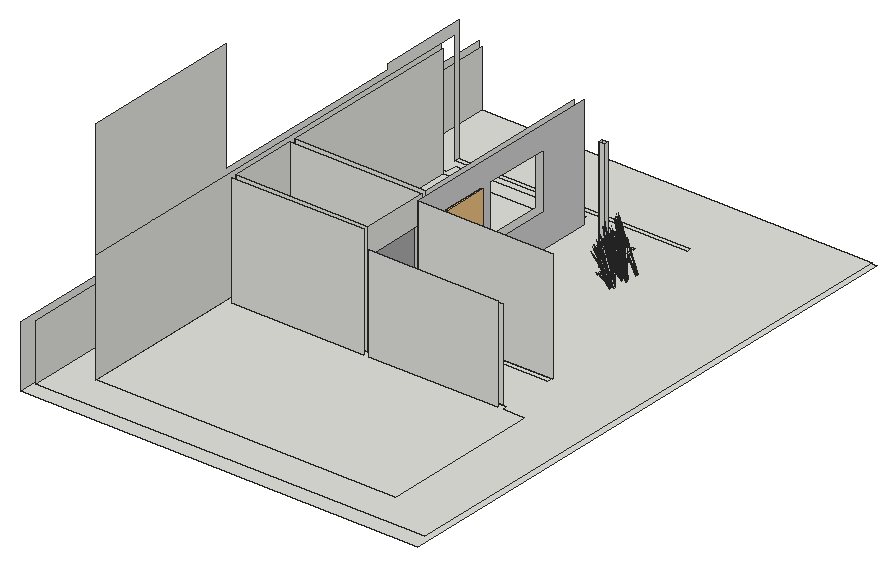
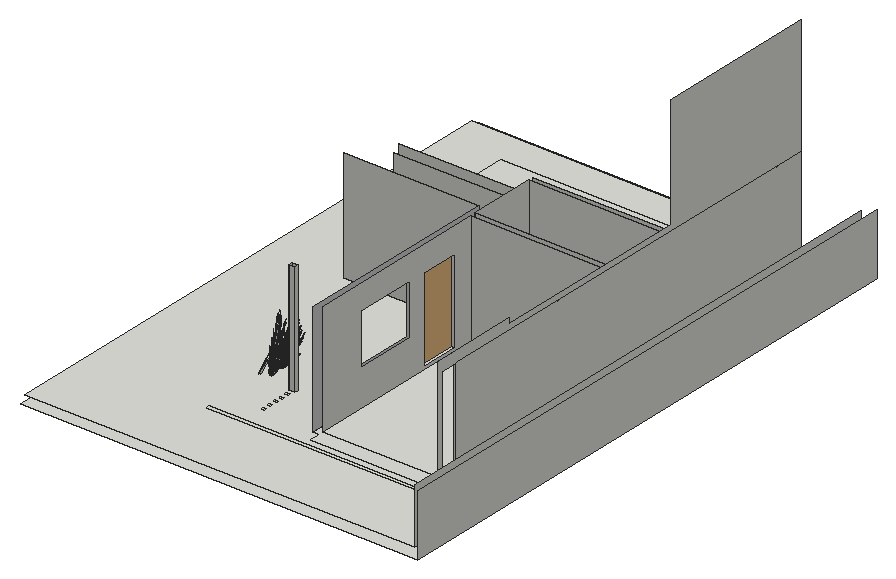
# SketchUp Ruby script. Lengths in inches.
U = 1.inch
M = Sketchup.active_model
def pt(a) = Geom::Point3d.new(a.map { |v| v * U })
def face(e, loops, mat)
  f = e.add_face(loops[0].map { |a| pt(a) })
  loops[1..].each { |l| e.add_face(l.map { |a| pt(a) }).erase! }
  f.material = f.back_material = mat if mat
  f
end
# faces: each face lists its corners as indices into pts; further lists are holes
def faces(e, pts, list, mat = nil) = list.each { |f| face(e, (f[0].is_a?(Array) ? f : [f]).map { |l| l.map { |i| pts[i] } }, mat) }
# xy, xz, yz: faces in a plane at the given z, y or x. An outline is a flat list of corners, or four numbers for a rectangle; further outlines are holes
def ring(l) = l.size == 4 ? [[l[0], l[1]], [l[2], l[1]], [l[2], l[3]], [l[0], l[3]]] : l.each_slice(2).to_a
def flat(e, list, mat, &to3) = list.each { |f| face(e, (f[0].is_a?(Array) ? f : [f]).map { |l| ring(l).map { |u, v| to3.(u, v) } }, mat) }
def xy(e, z, list, mat = nil) = flat(e, list, mat) { |x, y| [x, y, z] }
def xz(e, y, list, mat = nil) = flat(e, list, mat) { |x, z| [x, y, z] }
def yz(e, x, list, mat = nil) = flat(e, list, mat) { |y, z| [x, y, z] }
def lines(e, pts, list) = list.each { |a, b| e.add_line(pt(pts[a]), pt(pts[b])) }
# prism: a flat outline (further loops are holes) pulled along v
def prism(e, loops, v, mat = nil)
  f = face(e, loops, mat); d = Geom::Vector3d.new(v.map { |x| x * U })
  f.pushpull(f.normal.samedirection?(d) ? d.length : -d.length)
end
def box(e, o, s, mat = nil) = prism(e, [[o, [o[0] + s[0], o[1], o[2]], [o[0] + s[0], o[1] + s[1], o[2]], [o[0], o[1] + s[1], o[2]]]], [0, 0, s[2]], mat)
def at(x, y, z, deg = 0) = Geom::Transformation.translation(pt([x, y, z])) * Geom::Transformation.rotation(ORIGIN, Z_AXIS, deg.degrees)
def axes(o, x, y, z) = Geom::Transformation.new([*x, 0, *y, 0, *z, 0, *pt(o).to_a, 1])
def part(name) = M.definitions.add(name)
# library, detail: a bought-in or finely detailed component or shape, given as its bounding box
def library(name, o, s) = part(name).tap { |d| box(d.entities, o, s) }
def detail(e, o, s) = box(e.add_group.entities, o, s)
def put(e, d, t, mat = nil) = e.add_instance(d, t).tap { |i| i.material = mat if mat }
def group(e, t, mat = nil) = e.add_group.tap { |g| g.transformation = t; g.material = mat if mat }.entities
root = M.entities
M.materials.add("LightPink_Translucent").color = [144, 107, 117]
M.materials["LightPink_Translucent"].alpha = 0.75
M.materials.add("[0132_LightGray]").color = [169, 169, 169]
M.materials.add("[Cladding_Siding_White]1").color = [207, 207, 207]
c1 = library("porta+4",[0.2,-5.42,1.33],[46.55,4.72,83.21])
c2 = part("blade")
p = [[2.15,0.21,22],[0,0.17,0],[0.09,0.45,0],[2.18,0.31,22],[2.29,0.31,22],[0.38,0.45,0],
  [2.48,0.24,33],[2.49,0.24,33],[2.48,0.22,33]]
faces(c2.entities,p,[[0,1,2,3],[4,5,2,3],[6,3,4,7],[8,0,3,6]])
c3 = part("seeds")
p = [[0.3,-0.1,1.38],[-0.01,-0.03,1.59],[-0.01,-0.03,0.03],[0.14,-0.07,-0.07],[0.29,-0.03,3],[0.15,0.01,3.11]]
faces(c3.entities,p,[[0,1,2,3],[1,0,4,5]],"LightPink_Translucent")
c4 = part("blade with seeds")
put(c4.entities,c2,at(0,0,0))
put(c4.entities,c3,axes([2.4,0.25,30.99],[1.5799,-0.05474,1.17369],[-0.12525,1.92788,0.29478],[-0.07173,-0.02425,1.56792]))
xy(root,-6,[[0,0,426,612.89]])
xy(root,0,[[[9,9,426,606.89],[45,45,45,507,51,507,51,519,192,519,192,507,198,507,198,285,342,285,342,279,198,279,198,225,342,225,342,219,366,219,366,45],[45,525,294,531],[252,499,258,503],[252,491,258,495],[252,483,258,487],[252,475,258,479],[252,467,258,471],[252,459,258,463]],[51,225,192,297],[51,303,192,501]])
xy(root,3,[[192,324,198,366]])
xz(root,219,[[51,0,192,120],[198,0,336,102]])
xz(root,225,[[51,0,192,120],[198,0,336,96]])
xz(root,285,[[198,0,342,120]])
xz(root,297,[[51,0,192,120]])
xz(root,303,[[51,0,192,120]])
xz(root,324,[[192,3,198,93]])
xz(root,366,[[192,3,198,93]])
xz(root,459,[[252,0,258,120]])
xz(root,463,[[252,0,258,120]])
yz(root,0,[[0,-6,612.89,60]])
yz(root,9,[[9,0,606.89,60]])
yz(root,45,[[45,0,507,120],[525,0,525,120,45,120,45,246,219,246,219,126,435,126,435,132,531,132,531,0]])
yz(root,51,[[225,0,297,120],[303,0,501,120]])
yz(root,192,[[225,0,297,120],[[303,0,501,120],[324,3,366,93],[384,39,450,93]]])
yz(root,198,[[279,0,285,96],[[321,0,369,96],[324,3,366,93]]])
yz(root,198,[[225,0,279,96]],"[0132_LightGray]")
yz(root,198,[[[285,0,321,0,321,96,369,96,369,0,507,0,507,120,285,120],[381,36,453,96]]],"[Cladding_Siding_White]1")
yz(root,252,[[459,0,463,120]])
yz(root,258,[[459,0,463,120]])
put(root,c1,axes([195.24,320.8,-1.54],[0,1.02,0],[-1,0,0],[0,0,1.15408]))
put(root,c4,axes([282.74,451.66,3.875],[0.37107,-0.01478,1.71376],[-0.24616,0.64047,0.13857],[-0.5288,-0.03961,0.73262]))
put(root,c4,axes([282.9,452.79,3.875],[0.31041,-0.13801,1.71376],[0.26133,0.63772,0.13857],[-0.48731,0.14413,0.73262]))
put(root,c4,axes([281.93,453.875,2.59],[0.3109,0.05356,1.43002],[0.20038,0.54709,-0.30754],[-0.42231,0.10241,0.61141]))
put(root,c4,axes([284.68,452.125,3.34],[0.25429,-0.09438,1.77064],[0.08769,0.65901,0.13857],[-0.5508,0.08745,0.63284]))
put(root,c4,axes([284.1875,434.6,3.875],[0.37107,-0.01478,1.71376],[-0.24616,0.64047,0.13857],[-0.5288,-0.03961,0.73262]))
put(root,c4,axes([281.95,452.57,4.72],[-0.14609,0.08471,1.74944],[0.01243,0.61893,-0.27667],[-0.33486,0.08049,0.14031]))
put(root,c4,axes([283.85,451.07,4.98],[-0.89428,-0.01571,-0.71045],[0.06006,-0.66153,0.08574],[-0.37886,-0.06981,1.00501]))
put(root,c4,axes([283.13,451.23,2.59],[0.17466,0.18165,1.43002],[-0.40248,0.49377,-0.30754],[-0.41327,-0.11802,0.61141]))
put(root,c4,axes([282.42,452.21,4.53],[-0.74348,-0.18202,-0.35414],[0.21685,-0.53102,0.4572],[-0.29933,0.04869,0.87481]))
put(root,c4,axes([284.34,435.72,3.875],[0.31041,-0.13801,1.71376],[0.26133,0.63772,0.13857],[-0.48731,0.14413,0.73262]))
put(root,c4,axes([283.45,450.63,3.875],[0.3323,0.11241,1.71376],[-0.68769,0.4716,0.13857],[-0.42861,-0.21275,0.73262]))
put(root,c4,axes([283.375,436.81,2.59],[0.3109,0.05356,1.43002],[0.20038,0.54709,-0.30754],[-0.42231,0.10241,0.61141]))
put(root,c4,axes([280.33,453.19,4.71],[0.11417,0.0175,1.77383],[0.35319,0.57649,-0.16761],[-0.23371,0.15131,0.31391]))
put(root,c4,axes([282.93,452.48,4.68],[-0.24236,0.59349,-0.51099],[-0.83094,-0.20343,-0.3958],[-0.33455,0.05442,0.97773]))
put(root,c4,axes([283.56,451.2,4.68],[-0.6496,0.4322,-0.51099],[-0.5689,-0.45657,-0.3958],[-0.33005,-0.06576,0.97773]))
put(root,c4,axes([286.125,435.06,3.34],[0.25429,-0.09438,1.77064],[0.08769,0.65901,0.13857],[-0.5508,0.08745,0.63284]))
put(root,c4,axes([282.51,452.45,1.49],[0.02269,0.10283,1.76342],[-0.45738,0.53699,-0.26939],[-0.32488,-0.02707,0.30037]))
put(root,c4,axes([282.64,449.99,4.71],[0.06632,0.06511,1.77383],[-0.31973,0.58531,-0.16761],[-0.32381,0.00424,0.31391]))
put(root,c4,axes([281.28,455.02,2.77],[0.37283,-0.29571,1.1486],[0.14711,0.46813,0.84392],[-0.26943,0.08382,0.25299]))
put(root,c4,axes([283.38,449.6,4.72],[-0.19249,-0.00461,1.74944],[-0.61281,0.46055,-0.27667],[-0.32697,-0.0941,0.14031]))
put(root,c4,axes([283.39,435.5,4.72],[-0.14609,0.08471,1.74944],[0.01243,0.61893,-0.27667],[-0.33486,0.08049,0.14031]))
put(root,c4,axes([285.3,434,4.98],[-0.89428,-0.01571,-0.71045],[0.06006,-0.66153,0.08574],[-0.37886,-0.06981,1.00501]))
put(root,c4,axes([282.59,452.15,4.73],[0.25275,-0.59491,0.48003],[0.83094,0.20343,0.3958],[-0.32677,0.03575,0.9933]))
put(root,c4,axes([284.58,434.16,2.59],[0.17466,0.18165,1.43002],[-0.40248,0.49377,-0.30754],[-0.41327,-0.11802,0.61141]))
put(root,c4,axes([282.89,451.98,5.03],[0.45012,0.59081,-0.1216],[-0.79888,0.29033,-0.67495],[-0.33665,0.07795,1.02557]))
put(root,c4,axes([283.9,450.75,5.03],[-0.0479,0.66354,-0.1216],[-0.90696,-0.01814,-0.67495],[-0.3493,-0.04609,1.02557]))
put(root,c4,axes([283.32,450.79,4.53],[-0.50902,-0.40851,-0.35414],[0.58122,-0.38671,0.4572],[-0.29531,-0.05884,0.87481]))
put(root,c4,axes([282.53,451.99,4.73],[-0.32857,-0.44488,0.0643],[0.59916,-0.21775,0.50621],[-0.26412,0.04296,0.77189]))
put(root,c4,axes([283.86,435.15,4.53],[-0.74348,-0.18202,-0.35414],[0.21685,-0.53102,0.4572],[-0.29933,0.04869,0.87481]))
put(root,c4,axes([284.89,433.57,3.875],[0.3323,0.11241,1.71376],[-0.68769,0.4716,0.13857],[-0.42861,-0.21275,0.73262]))
put(root,c4,axes([284.03,453.22,3.875],[0.22344,-0.20048,1.71376],[0.56419,0.54113,0.13857],[-0.38697,0.24643,0.73262]))
put(root,c4,axes([282.69,453.74,4.53],[-0.77872,0.09325,-0.35414],[-0.20563,-0.53305,0.4572],[-0.22316,0.14318,0.87481]))
put(root,c4,axes([282.27,455.33,1.49],[0.12,0.06519,1.76342],[0.20347,0.60397,-0.26939],[-0.26596,0.12879,0.30037]))
put(root,c4,axes([282.09,451.77,2.77],[0.57115,-0.04669,1.1486],[-0.36229,0.41137,0.84392],[-0.28224,-0.06171,0.25299]))
put(root,c4,axes([281.77,436.125,4.71],[0.11417,0.0175,1.77383],[0.35319,0.57649,-0.16761],[-0.23371,0.15131,0.31391]))
put(root,c4,axes([284.37,435.42,4.68],[-0.24236,0.59349,-0.51099],[-0.83094,-0.20343,-0.3958],[-0.33455,0.05442,0.97773]))
put(root,c4,axes([285,434.13,4.68],[-0.6496,0.4322,-0.51099],[-0.5689,-0.45657,-0.3958],[-0.33005,-0.06576,0.97773]))
put(root,c4,axes([282.79,453.63,4.73],[-0.22187,-0.60049,0.48003],[0.87033,-0.10422,0.3958],[-0.25651,0.14123,0.9933]))
put(root,c4,axes([283.95,435.38,1.49],[0.02269,0.10283,1.76342],[-0.45738,0.53699,-0.26939],[-0.32488,-0.02707,0.30037]))
put(root,c4,axes([283.24,450.64,5.09],[0.7388,-0.48151,0.53763],[0.63717,0.51135,0.4433],[-0.34662,-0.08882,1.11249]))
put(root,c4,axes([282.62,453.51,4.73],[-0.61415,-0.2744,0.0643],[0.35756,-0.39076,0.50621],[-0.1969,0.12633,0.77189]))
put(root,c4,axes([284.08,432.92,4.71],[0.06632,0.06511,1.77383],[-0.31973,0.58531,-0.16761],[-0.32381,0.00424,0.31391]))
put(root,c4,axes([282.73,437.96,2.77],[0.37283,-0.29571,1.1486],[0.14711,0.46813,0.84392],[-0.26943,0.08382,0.25299]))
put(root,c4,axes([284.82,432.53,4.72],[-0.19249,-0.00461,1.74944],[-0.61281,0.46055,-0.27667],[-0.32697,-0.0941,0.14031]))
put(root,c4,axes([283.87,453.71,3.875],[0.16657,-0.22426,1.71376],[0.69879,0.4641,0.13857],[-0.31524,0.28926,0.73262]))
put(root,c4,axes([284.03,435.08,4.73],[0.25275,-0.59491,0.48003],[0.83094,0.20343,0.3958],[-0.32677,0.03575,0.9933]))
put(root,c4,axes([284.33,434.91,5.03],[0.45012,0.59081,-0.1216],[-0.79888,0.29033,-0.67495],[-0.33665,0.07795,1.02557]))
put(root,c4,axes([285.34,433.68,5.03],[-0.0479,0.66354,-0.1216],[-0.90696,-0.01814,-0.67495],[-0.3493,-0.04609,1.02557]))
put(root,c4,axes([284.76,433.73,4.53],[-0.50902,-0.40851,-0.35414],[0.58122,-0.38671,0.4572],[-0.29531,-0.05884,0.87481]))
put(root,c4,axes([283.2,452.15,5.05],[0.74348,0.18202,0.35414],[-0.21685,0.53102,-0.4572],[-0.29933,0.04869,0.87481]))
put(root,c4,axes([283.97,434.92,4.73],[-0.32857,-0.44488,0.0643],[0.59916,-0.21775,0.50621],[-0.26412,0.04296,0.77189]))
put(root,c4,axes([285.48,436.15,3.875],[0.22344,-0.20048,1.71376],[0.56419,0.54113,0.13857],[-0.38697,0.24643,0.73262]))
put(root,c4,axes([284.13,436.68,4.53],[-0.77872,0.09325,-0.35414],[-0.20563,-0.53305,0.4572],[-0.22316,0.14318,0.87481]))
put(root,c4,axes([283.33,453.81,4.68],[0.22982,0.59576,-0.51099],[-0.87033,0.10422,-0.3958],[-0.24941,0.16002,0.97773]))
put(root,c4,axes([283.58,450.64,4.73],[0.04505,-0.49615,0.0643],[0.68022,0.0136,0.50621],[-0.26056,-0.05192,0.77189]))
put(root,c4,axes([281.97,454.875,4.72],[-0.02224,0.12912,1.74944],[0.63107,0.44917,-0.27667],[-0.16521,0.21241,0.14031]))
put(root,c4,axes([283.71,438.26,1.49],[0.12,0.06519,1.76342],[0.20347,0.60397,-0.26939],[-0.26596,0.12879,0.30037]))
put(root,c4,axes([285.5,453.38,2.06],[-0.9306,-0.10697,-0.62353],[0.19638,-0.65984,-0.16365],[-0.27771,-0.07995,1.37633]))
put(root,c4,axes([283.54,434.71,2.77],[0.57115,-0.04669,1.1486],[-0.36229,0.41137,0.84392],[-0.28224,-0.06171,0.25299]))
put(root,c4,axes([285.67,449.78,5.43],[-0.59706,0.6255,-0.13619],[-0.86465,-0.36036,-0.75594],[-0.30056,-0.17672,1.14864]))
put(root,c4,axes([284.04,451.01,5.05],[0.50902,0.40851,0.35414],[-0.58122,0.38671,-0.4572],[-0.29531,-0.05884,0.87481]))
put(root,c4,axes([285.41,450.29,4.98],[-0.76283,-0.31537,-0.71045],[0.54213,-0.55263,0.08574],[-0.27638,-0.1883,1.00501]))
put(root,c4,axes([284.23,436.5625,4.73],[-0.22187,-0.60049,0.48003],[0.87033,-0.10422,0.3958],[-0.25651,0.14123,0.9933]))
put(root,c4,axes([285.05,450.3,4.68],[-0.88277,0.1551,-0.51099],[-0.15442,-0.58737,-0.3958],[-0.23711,-0.16832,0.97773]))
put(root,c4,axes([284.68,433.57,5.09],[0.7388,-0.48151,0.53763],[0.63717,0.51135,0.4433],[-0.34662,-0.08882,1.11249]))
put(root,c4,axes([284.0625,436.45,4.73],[-0.61415,-0.2744,0.0643],[0.35756,-0.39076,0.50621],[-0.1969,0.12633,0.77189]))
put(root,c4,axes([284.28,454.63,2.02],[-0.83726,-0.32623,-0.49651],[0.50045,-0.58498,0],[-0.19069,-0.0743,1.57504]))
put(root,c4,axes([283.91,449.77,1.49],[-0.08666,0.08595,1.76342],[-0.87574,0.18531,-0.26939],[-0.21156,-0.16858,0.30037]))
put(root,c4,axes([282.92,453.38,5.03],[0.82753,0.35977,-0.1216],[-0.47675,0.52101,-0.67495],[-0.2338,0.18111,1.02557]))
put(root,c4,axes([284.79,455.02,2.375],[-0.55932,0.6538,0],[-0.93577,-0.36461,-0.51607],[-0.21313,-0.08304,1.63711]))
put(root,c4,axes([285.31,436.65,3.875],[0.16657,-0.22426,1.71376],[0.69879,0.4641,0.13857],[-0.31524,0.28926,0.73262]))
put(root,c4,axes([284.64,435.09,5.05],[0.74348,0.18202,0.35414],[-0.21685,0.53102,-0.4572],[-0.29933,0.04869,0.87481]))
put(root,c4,axes([281.56,454.94,5.65],[0.78943,0.17416,-0.06488],[-0.24284,0.53604,-0.29416],[-0.12912,0.08139,0.97024]))
put(root,c4,axes([284.77,436.74,4.68],[0.22982,0.59576,-0.51099],[-0.87033,0.10422,-0.3958],[-0.24941,0.16002,0.97773]))
put(root,c4,axes([283.33,453.43,5.05],[0.77872,-0.09325,0.35414],[0.20563,0.53305,-0.4572],[-0.22316,0.14318,0.87481]))
put(root,c4,axes([285.02,433.57,4.73],[0.04505,-0.49615,0.0643],[0.68022,0.0136,0.50621],[-0.26056,-0.05192,0.77189]))
put(root,c4,axes([283.42,437.81,4.72],[-0.02224,0.12912,1.74944],[0.63107,0.44917,-0.27667],[-0.16521,0.21241,0.14031]))
put(root,c4,axes([283.77,455.97,2.59],[0.28231,-0.10293,1.43002],[0.69701,0.31035,-0.30754],[-0.20746,0.26854,0.61141]))
put(root,c4,axes([286.94,436.3125,2.06],[-0.9306,-0.10697,-0.62353],[0.19638,-0.65984,-0.16365],[-0.27771,-0.07995,1.37633]))
put(root,c4,axes([287.11,432.71,5.43],[-0.59706,0.6255,-0.13619],[-0.86465,-0.36036,-0.75594],[-0.30056,-0.17672,1.14864]))
put(root,c4,axes([283.37,450.1,2.13],[-0.25807,0.53277,-0.03893],[-0.79428,-0.16389,-0.17649],[-0.1206,-0.08714,0.58215]))
put(root,c4,axes([285.48,433.94,5.05],[0.50902,0.40851,0.35414],[-0.58122,0.38671,-0.4572],[-0.29531,-0.05884,0.87481]))
put(root,c4,axes([285.4375,448.29,4.71],[-0.01669,0.07821,1.77383],[-0.82314,0.28383,-0.16761],[-0.24223,-0.14508,0.31391]))
put(root,c4,axes([286.85,433.22,4.98],[-0.76283,-0.31537,-0.71045],[0.54213,-0.55263,0.08574],[-0.27638,-0.1883,1.00501]))
put(root,c4,axes([286.5,433.24,4.68],[-0.88277,0.1551,-0.51099],[-0.15442,-0.58737,-0.3958],[-0.23711,-0.16832,0.97773]))
put(root,c4,axes([284.56,449.43,2.59],[-0.05417,0.21344,1.43002],[-0.79196,0.17867,-0.30754],[-0.18512,-0.27588,0.61141]))
put(root,c4,axes([284.82,449.98,3.875],[0.2045,0.20949,1.71376],[-0.94495,0.17636,0.13857],[-0.21357,-0.32887,0.73262]))
put(root,c4,axes([286.56,453.48,2.67],[-0.90324,0.43318,-0.29095],[-0.60064,-0.61207,-0.50002],[-0.22285,-0.06216,1.59708]))
put(root,c4,axes([284.0625,454.84,4.73],[-0.63704,-0.44518,0.48003],[0.67652,-0.38394,0.3958],[-0.11751,0.20886,0.9933]))
put(root,c4,axes([285.72,437.56,2.02],[-0.83726,-0.32623,-0.49651],[0.50045,-0.58498,0],[-0.19069,-0.0743,1.57504]))
put(root,c4,axes([285.36,432.7,1.49],[-0.08666,0.08595,1.76342],[-0.87574,0.18531,-0.26939],[-0.21156,-0.16858,0.30037]))
put(root,c4,axes([284.36,436.3125,5.03],[0.82753,0.35977,-0.1216],[-0.47675,0.52101,-0.67495],[-0.2338,0.18111,1.02557]))
put(root,c4,axes([285.15,449.87,4.53],[-0.13817,-0.52554,-0.35414],[0.78985,-0.13877,0.4572],[-0.21215,-0.1506,0.87481]))
put(root,c4,axes([282.94,452.53,2.375],[-1.11865,0,0],[0,-0.72922,-0.51607],[0,-0.16609,1.63711]))
put(root,c4,axes([284.51,454.38,2.03],[-0.21015,-0.56852,-0.30978],[0.83462,-0.16144,0.30978],[-0.16826,-0.06556,1.38974]))
put(root,c4,axes([290.44,446.43,3.875],[0.37107,-0.01478,1.71376],[-0.24616,0.64047,0.13857],[-0.5288,-0.03961,0.73262]))
put(root,c4,axes([290.45,461.1,3.875],[0.37107,-0.01478,1.71376],[-0.24616,0.64047,0.13857],[-0.5288,-0.03961,0.73262]))
put(root,c4,axes([286.23,437.95,2.375],[-0.55932,0.6538,0],[-0.93577,-0.36461,-0.51607],[-0.21313,-0.08304,1.63711]))
put(root,c4,axes([283.83,454.8,4.73],[-0.73517,-0.0304,0.0643],[0.02016,-0.45906,0.50621],[-0.07693,0.17585,0.77189]))
put(root,c4,axes([284.06,454.98,4.53],[-0.60531,0.34352,-0.35414],[-0.573,-0.39225,0.4572],[-0.08718,0.19929,0.87481]))
put(root,c4,axes([283,437.875,5.65],[0.78943,0.17416,-0.06488],[-0.24284,0.53604,-0.29416],[-0.12912,0.08139,0.97024]))
put(root,c4,axes([287.16,453.95,2.06],[-0.60257,0.49041,-0.62353],[-0.74854,-0.44469,-0.16365],[-0.24146,0.12234,1.37633]))
put(root,c4,axes([285.61,450.3,5.05],[0.13817,0.52554,0.35414],[-0.78985,0.13877,-0.4572],[-0.21215,-0.1506,0.87481]))
put(root,c4,axes([281.9,456.2,4.71],[0.10149,-0.03939,1.77383],[0.83886,0.26202,-0.16761],[-0.01971,0.21816,0.31391]))
put(root,c4,axes([284.77,436.36,5.05],[0.77872,-0.09325,0.35414],[0.20563,0.53305,-0.4572],[-0.22316,0.14318,0.87481]))
put(root,c4,axes([283.81,452.34,2.33],[-0.83213,0.54855,0.30756],[-0.83263,-0.54278,-0.36492],[-0.02906,-0.15578,1.64885]))
put(root,c4,axes([285.21,438.9,2.59],[0.28231,-0.10293,1.43002],[0.69701,0.31035,-0.30754],[-0.20746,0.26854,0.61141]))
put(root,c4,axes([287.24,453.85,3.33],[0.77308,0.2631,1.51261],[-0.75736,0.56681,0.59816],[-0.33924,-0.33594,1.26806]))
put(root,c4,axes([284.8125,433.03,2.13],[-0.25807,0.53277,-0.03893],[-0.79428,-0.16389,-0.17649],[-0.1206,-0.08714,0.58215]))
put(root,c4,axes([284.28,449.08,2.77],[0.46666,0.22709,1.1486],[-0.67962,0.13651,0.84392],[-0.14541,-0.17452,0.25299]))
put(root,c4,axes([287.57,453.67,2.46],[-0.87356,-0.52515,-0.25192],[0.73507,-0.5897,0.5513],[-0.23523,0.06143,1.68216]))
put(root,c4,axes([285.98,453.17,2.21],[-0.53742,-0.54764,-0.44739],[0.81403,-0.38564,0.21531],[-0.17391,-0.06776,1.43643]))
put(root,c4,axes([290.59,447.55,3.875],[0.31041,-0.13801,1.71376],[0.26133,0.63772,0.13857],[-0.48731,0.14413,0.73262]))
put(root,c4,axes([290.61,462.23,3.875],[0.31041,-0.13801,1.71376],[0.26133,0.63772,0.13857],[-0.48731,0.14413,0.73262]))
